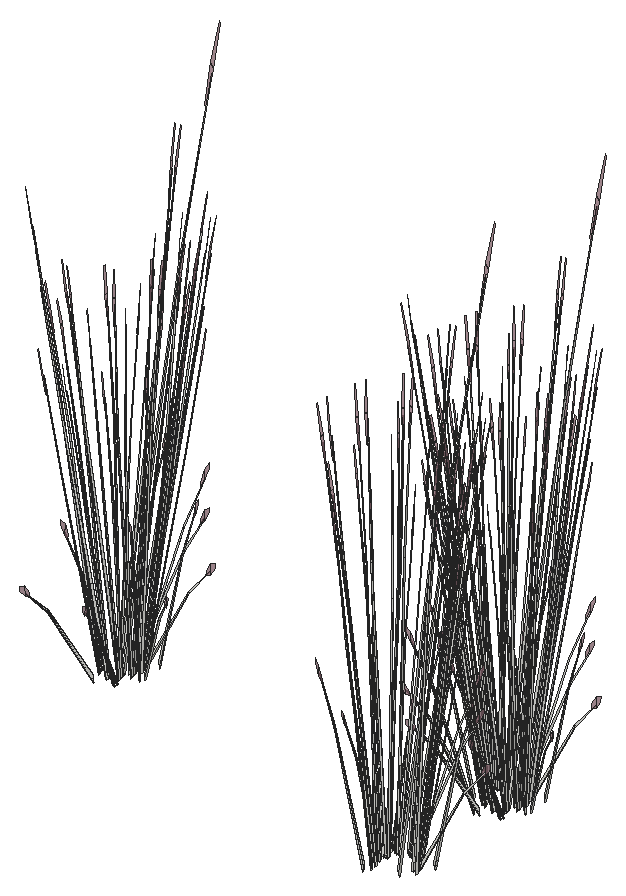
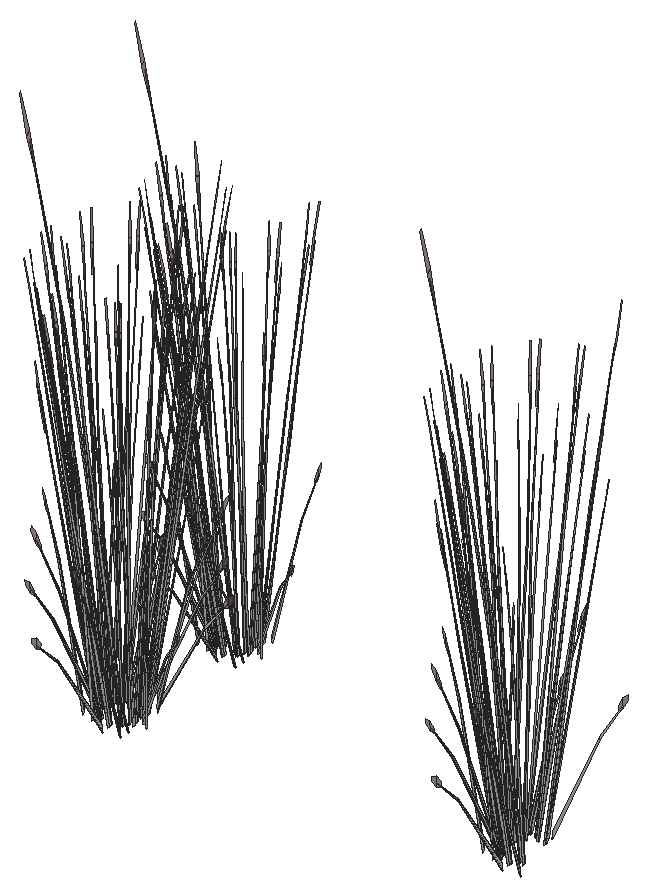
# SketchUp Ruby script. Lengths in inches.
U = 1.inch
M = Sketchup.active_model
def pt(a) = Geom::Point3d.new(a.map { |v| v * U })
def face(e, loops, mat)
  f = e.add_face(loops[0].map { |a| pt(a) })
  loops[1..].each { |l| e.add_face(l.map { |a| pt(a) }).erase! }
  f.material = f.back_material = mat if mat
  f
end
# faces: each face lists its corners as indices into pts; further lists are holes
def faces(e, pts, list, mat = nil) = list.each { |f| face(e, (f[0].is_a?(Array) ? f : [f]).map { |l| l.map { |i| pts[i] } }, mat) }
# xy, xz, yz: faces in a plane at the given z, y or x. An outline is a flat list of corners, or four numbers for a rectangle; further outlines are holes
def ring(l) = l.size == 4 ? [[l[0], l[1]], [l[2], l[1]], [l[2], l[3]], [l[0], l[3]]] : l.each_slice(2).to_a
def flat(e, list, mat, &to3) = list.each { |f| face(e, (f[0].is_a?(Array) ? f : [f]).map { |l| ring(l).map { |u, v| to3.(u, v) } }, mat) }
def xy(e, z, list, mat = nil) = flat(e, list, mat) { |x, y| [x, y, z] }
def xz(e, y, list, mat = nil) = flat(e, list, mat) { |x, z| [x, y, z] }
def yz(e, x, list, mat = nil) = flat(e, list, mat) { |y, z| [x, y, z] }
def lines(e, pts, list) = list.each { |a, b| e.add_line(pt(pts[a]), pt(pts[b])) }
# prism: a flat outline (further loops are holes) pulled along v
def prism(e, loops, v, mat = nil)
  f = face(e, loops, mat); d = Geom::Vector3d.new(v.map { |x| x * U })
  f.pushpull(f.normal.samedirection?(d) ? d.length : -d.length)
end
def box(e, o, s, mat = nil) = prism(e, [[o, [o[0] + s[0], o[1], o[2]], [o[0] + s[0], o[1] + s[1], o[2]], [o[0], o[1] + s[1], o[2]]]], [0, 0, s[2]], mat)
def at(x, y, z, deg = 0) = Geom::Transformation.translation(pt([x, y, z])) * Geom::Transformation.rotation(ORIGIN, Z_AXIS, deg.degrees)
def axes(o, x, y, z) = Geom::Transformation.new([*x, 0, *y, 0, *z, 0, *pt(o).to_a, 1])
def part(name) = M.definitions.add(name)
# library, detail: a bought-in or finely detailed component or shape, given as its bounding box
def library(name, o, s) = part(name).tap { |d| box(d.entities, o, s) }
def detail(e, o, s) = box(e.add_group.entities, o, s)
def put(e, d, t, mat = nil) = e.add_instance(d, t).tap { |i| i.material = mat if mat }
def group(e, t, mat = nil) = e.add_group.tap { |g| g.transformation = t; g.material = mat if mat }.entities
root = M.entities
M.materials.add("LightPink_Translucent").color = [144, 107, 117]
M.materials["LightPink_Translucent"].alpha = 0.75
c1 = part("blade")
p = [[2.15,0.21,22],[0,0.17,0],[0.09,0.45,0],[2.18,0.31,22],[2.29,0.31,22],[0.38,0.45,0],
  [2.48,0.24,33],[2.49,0.24,33],[2.48,0.22,33]]
faces(c1.entities,p,[[0,1,2,3],[4,5,2,3],[6,3,4,7],[8,0,3,6]])
c2 = part("seeds")
p = [[0.3,-0.1,1.38],[-0.01,-0.03,1.59],[-0.01,-0.03,0.03],[0.14,-0.07,-0.07],[0.29,-0.03,3],[0.15,0.01,3.11]]
faces(c2.entities,p,[[0,1,2,3],[1,0,4,5]],"LightPink_Translucent")
c3 = part("blade with seeds")
put(c3.entities,c1,at(0,0,0))
put(c3.entities,c2,axes([2.4,0.25,30.99],[1.5799,-0.05474,1.17369],[-0.12525,1.92788,0.29478],[-0.07173,-0.02425,1.56792]))
put(root,c3,axes([366.93,790.19,4.73],[-0.29004,-0.02173,0.0643],[0.00795,-0.32812,0.50621],[-0.03035,0.12569,0.77189]))
put(root,c3,axes([367.63,786.97,5.05],[0.05451,0.37564,0.35414],[-0.31161,0.09919,-0.4572],[-0.0837,-0.10765,0.87481]))
put(root,c3,axes([366.17,791.1875,4.71],[0.04004,-0.02816,1.77383],[0.33095,0.18728,-0.16761],[-0.00778,0.15594,0.31391]))
put(root,c3,axes([367.49,786.53,5.09],[0.39316,-0.11987,0.53763],[0.06823,0.47021,0.4433],[-0.09247,-0.13858,1.11249]))
put(root,c3,axes([367.58,786.63,4.73],[0.16041,-0.29625,0.0643],[0.22843,0.17248,0.50621],[-0.07385,-0.09498,0.77189]))
put(root,c3,axes([367.94,785.75,4.72],[-0.05398,-0.06539,1.74944],[-0.36026,0.04145,-0.27667],[-0.0575,-0.15639,0.14031]))
put(root,c3,axes([367.15,789.97,5.05],[0.23881,-0.24554,0.35414],[0.22606,0.28036,-0.4572],[-0.0344,0.14245,0.87481]))
put(root,c3,axes([366.99,790.03,5.4],[0.3879,0.02311,-0.13498],[-0.0106,0.43749,-0.74919],[-0.02694,0.1685,1.13838]))
put(root,c3,axes([368.48,786.76,5.03],[-0.34538,0.21713,-0.1216],[-0.16972,-0.38536,-0.67495],[-0.04557,-0.16239,1.02557]))
put(root,c3,axes([368.38,786.91,5.05],[-0.1064,0.35863,0.35414],[-0.31043,-0.1046,-0.4572],[-0.02846,-0.14439,0.87481]))
put(root,c3,axes([367.8125,790.67,5.0625],[-0.34777,-0.12192,0.53283],[0.11892,-0.40083,0.43934],[0.0209,0.15763,1.10256]))
put(root,c3,axes([367.72,790.7,4.73],[-0.26007,0.1585,0.0643],[-0.12729,-0.28902,0.50621],[0.02512,0.1274,0.77189]))
put(root,c3,axes([368.48,786.59,4.73],[0.26007,-0.1585,0.0643],[0.12729,0.28902,0.50621],[-0.02512,-0.1274,0.77189]))
put(root,c3,axes([367.63,791.38,4.72],[0.04474,0.0751,1.74944],[0.36104,0.0295,-0.27667],[0.03631,0.16562,0.14031]))
put(root,c3,axes([368.38,786.62,4.73],[0.34777,0.12192,0.48003],[-0.11892,0.40083,0.3958],[-0.0209,-0.15763,0.9933]))
put(root,c3,axes([367.82,790.37,5.05],[0.1064,-0.35863,0.35414],[0.31043,0.1046,-0.4572],[0.02846,0.14439,0.87481]))
put(root,c3,axes([368.23,791.65,5.65],[0.2439,-0.26754,-0.06488],[0.22348,0.29302,-0.29416],[0.01573,0.08303,0.97024]))
put(root,c3,axes([367.71,790.52,5.03],[0.34538,-0.21713,-0.1216],[0.16972,0.38536,-0.67495],[0.04557,0.16239,1.02557]))
put(root,c3,axes([369.48,786.22,4.71],[-0.03584,0.03562,1.77383],[-0.35118,-0.12018,-0.16761],[-0.01271,-0.15545,0.31391]))
put(root,c3,axes([369.2,787.25,5.03],[-0.3879,-0.02311,-0.1216],[0.0106,-0.43749,-0.67495],[0.02694,-0.1685,1.02557]))
put(root,c3,axes([369.05,787.32,5.05],[-0.23881,0.24554,0.35414],[-0.22606,-0.28036,-0.4572],[0.0344,-0.14245,0.87481]))
put(root,c3,axes([368.68,790.57,4.73],[-0.35104,0.10702,0.48003],[-0.06092,-0.41983,0.3958],[0.08256,0.12373,0.9933]))
put(root,c3,axes([368.61,790.65,4.73],[-0.16041,0.29625,0.0643],[-0.22843,-0.17248,0.50621],[0.07385,0.09498,0.77189]))
put(root,c3,axes([368.5625,790.3125,5.05],[-0.05451,-0.37564,0.35414],[0.31161,-0.09919,-0.4572],[0.0837,0.10765,0.87481]))
put(root,c3,axes([368.77,788.15,4.47],[-0.30498,-0.24231,1.38283],[0.32203,-0.37727,0.59665],[0.0984,0.22736,1.33663]))
put(root,c3,axes([368.26,790.84,4.71],[0.00104,-0.05646,1.77383],[0.30246,-0.2491,-0.16761],[0.10506,0.08891,0.31391]))
put(root,c3,axes([369.27,787.09,4.73],[0.29004,0.02173,0.0643],[-0.00795,0.32812,0.50621],[0.03035,-0.12569,0.77189]))
put(root,c3,axes([369.55,786.55,4.72],[-0.00341,-0.09282,1.74944],[-0.28775,-0.26825,-0.27667],[0.04449,-0.16261,0.14031]))
put(root,c3,axes([369.17,787.0625,4.73],[0.25132,0.3182,0.48003],[-0.2669,0.27442,0.3958],[0.04636,-0.14929,0.9933]))
put(root,c3,axes([369.46,788.07,5.05],[-0.30722,0.06665,0.35414],[-0.08112,-0.381,-0.4572],[0.08804,-0.10234,0.87481]))
put(root,c3,axes([368.53,790.51,5.03],[0.21031,-0.39918,-0.1216],[0.30457,0.22997,-0.67495],[0.10587,0.11278,1.02557]))
put(root,c3,axes([369.62,788.11,5.03],[-0.32648,-0.25715,-0.1216],[0.18809,-0.3724,-0.67495],[0.09224,-0.12945,1.02557]))
put(root,c3,axes([369.18,789.8,5.05],[-0.20082,-0.29199,0.35414],[0.2293,-0.2764,-0.4572],[0.1165,0.04206,0.87481]))
put(root,c3,axes([369.36,790.07,4.73],[-0.01777,0.35463,0.0643],[-0.26836,-0.00972,0.50621],[0.1028,0.03711,0.77189]))
put(root,c3,axes([369.39,789.96,4.73],[-0.26024,0.30729,0.48003],[-0.22444,-0.32634,0.3958],[0.1221,0.05668,0.9933]))
put(root,c3,axes([369.51,788.99,5.05],[-0.29332,-0.1301,0.35414],[0.08555,-0.37955,-0.4572],[0.11809,-0.0348,0.87481]))
put(root,c3,axes([369.74,788.01,4.73],[0.2423,0.19613,0.0643],[-0.14107,0.2793,0.50621],[0.07768,-0.0903,0.77189]))
put(root,c3,axes([369.67,787.93,4.73],[0.08753,0.42921,0.48003],[-0.34336,0.07449,0.3958],[0.1012,-0.10094,0.9933]))
put(root,c3,axes([370.43,788,4.71],[-0.0461,-0.00354,1.77383],[-0.19143,-0.37951,-0.16761],[0.07688,-0.12478,0.31391]))
put(root,c3,axes([369.78,789.1,4.73],[0.12963,0.31798,0.0643],[-0.23638,0.15564,0.50621],[0.1042,-0.03071,0.77189]))
put(root,c3,axes([369.24,789.99,5.03],[0.0189,-0.47427,-0.1216],[0.35781,0.01296,-0.67495],[0.13781,0.03295,1.02557]))
put(root,c3,axes([369.64,789.11,5.03],[-0.17758,-0.42229,-0.1216],[0.31518,-0.20752,-0.67495],[0.13282,-0.05572,1.02557]))
put(root,c3,axes([369.75,788.99,4.73],[-0.09971,0.42522,0.48003],[-0.32782,-0.1454,0.3958],[0.12892,-0.02555,0.9933]))
put(root,c3,axes([369.55,789.71,4.72],[0.07571,-0.00789,1.74944],[0.20767,-0.36231,-0.27667],[0.13467,0.04783,0.14031]))
put(root,c3,axes([370.34,790.37,4.71],[-0.03191,-0.04083,1.77383],[0.06981,-0.43764,-0.16761],[0.12571,-0.02796,0.31391]))
put(root,c3,axes([370.6,788.45,4.72],[0.04898,-0.07104,1.74944],[-0.06269,-0.43574,-0.27667],[0.12289,-0.08262,0.14031]))
put(root,c3,axes([400.14,777.88,4.72],[-0.05763,0.06055,1.74944],[0.0049,0.44239,-0.27667],[-0.13211,0.05753,0.14031]))
put(root,c3,axes([400.14,790.65,4.72],[-0.05763,0.06055,1.74944],[0.0049,0.44239,-0.27667],[-0.13211,0.05753,0.14031]))
put(root,c3,axes([399.5,778.33,4.71],[0.04504,0.01251,1.77383],[0.13934,0.41205,-0.16761],[-0.0922,0.10815,0.31391]))
put(root,c3,axes([399.5,791.1,4.71],[0.04504,0.01251,1.77383],[0.13934,0.41205,-0.16761],[-0.0922,0.10815,0.31391]))
put(root,c3,axes([400.42,776.04,4.71],[0.02617,0.04654,1.77383],[-0.12614,0.41836,-0.16761],[-0.12775,0.00303,0.31391]))
put(root,c3,axes([400.42,788.81,4.71],[0.02617,0.04654,1.77383],[-0.12614,0.41836,-0.16761],[-0.12775,0.00303,0.31391]))
put(root,c3,axes([400.71,788.53,4.72],[-0.07594,-0.00329,1.74944],[-0.24177,0.32918,-0.27667],[-0.129,-0.06726,0.14031]))
put(root,c3,axes([400.4,777.58,4.73],[0.09971,-0.42522,0.48003],[0.32782,0.1454,0.3958],[-0.12892,0.02555,0.9933]))
put(root,c3,axes([400.4,790.35,4.73],[0.09971,-0.42522,0.48003],[0.32782,0.1454,0.3958],[-0.12892,0.02555,0.9933]))
put(root,c3,axes([400.51,777.46,5.03],[0.17758,0.42229,-0.1216],[-0.31518,0.20752,-0.67495],[-0.13282,0.05572,1.02557]))
put(root,c3,axes([400.51,790.23,5.03],[0.17758,0.42229,-0.1216],[-0.31518,0.20752,-0.67495],[-0.13282,0.05572,1.02557]))
put(root,c3,axes([400.91,776.58,5.03],[-0.0189,0.47427,-0.1216],[-0.35781,-0.01296,-0.67495],[-0.13781,-0.03295,1.02557]))
put(root,c3,axes([400.91,789.35,5.03],[-0.0189,0.47427,-0.1216],[-0.35781,-0.01296,-0.67495],[-0.13781,-0.03295,1.02557]))
put(root,c3,axes([400.37,777.47,4.73],[-0.12963,-0.31798,0.0643],[0.23638,-0.15564,0.50621],[-0.1042,0.03071,0.77189]))
put(root,c3,axes([400.37,790.24,4.73],[-0.12963,-0.31798,0.0643],[0.23638,-0.15564,0.50621],[-0.1042,0.03071,0.77189]))
put(root,c3,axes([400.47,778.64,4.73],[-0.08753,-0.42921,0.48003],[0.34336,-0.07449,0.3958],[-0.1012,0.10094,0.9933]))
put(root,c3,axes([400.47,791.41,4.73],[-0.08753,-0.42921,0.48003],[0.34336,-0.07449,0.3958],[-0.1012,0.10094,0.9933]))
put(root,c3,axes([400.65,789.27,5.09],[0.29147,-0.34417,0.53763],[0.25138,0.3655,0.4433],[-0.13675,-0.06349,1.11249]))
put(root,c3,axes([400.41,778.56,4.73],[-0.2423,-0.19613,0.0643],[0.14107,-0.2793,0.50621],[-0.07768,0.0903,0.77189]))
put(root,c3,axes([400.41,791.33,4.73],[-0.2423,-0.19613,0.0643],[0.14107,-0.2793,0.50621],[-0.07768,0.0903,0.77189]))
put(root,c3,axes([400.64,777.59,5.05],[0.29332,0.1301,0.35414],[-0.08555,0.37955,-0.4572],[-0.11809,0.0348,0.87481]))
put(root,c3,axes([400.64,790.35,5.05],[0.29332,0.1301,0.35414],[-0.08555,0.37955,-0.4572],[-0.11809,0.0348,0.87481]))
put(root,c3,axes([400.78,789.27,4.73],[0.01777,-0.35463,0.0643],[0.26836,0.00972,0.50621],[-0.1028,-0.03711,0.77189]))
put(root,c3,axes([400.15,779.53,4.72],[-0.00877,0.09229,1.74944],[0.24897,0.32105,-0.27667],[-0.06518,0.15182,0.14031]))
put(root,c3,axes([400.15,792.3,4.72],[-0.00877,0.09229,1.74944],[0.24897,0.32105,-0.27667],[-0.06518,0.15182,0.14031]))
put(root,c3,axes([401.61,788.66,5.43],[-0.23555,0.44708,-0.13619],[-0.34112,-0.25757,-0.75594],[-0.11858,-0.12631,1.14864]))
put(root,c3,axes([400.97,776.77,5.05],[0.20082,0.29199,0.35414],[-0.2293,0.2764,-0.4572],[-0.1165,-0.04206,0.87481]))
put(root,c3,axes([400.97,789.54,5.05],[0.20082,0.29199,0.35414],[-0.2293,0.2764,-0.4572],[-0.1165,-0.04206,0.87481]))
put(root,c3,axes([400.53,778.46,5.03],[0.32648,0.25715,-0.1216],[-0.18809,0.3724,-0.67495],[-0.09224,0.12945,1.02557]))
put(root,c3,axes([400.53,791.23,5.03],[0.32648,0.25715,-0.1216],[-0.18809,0.3724,-0.67495],[-0.09224,0.12945,1.02557]))
put(root,c3,axes([399.99,779.58,5.65],[0.31145,0.12449,-0.06488],[-0.0958,0.38314,-0.29416],[-0.05094,0.05817,0.97024]))
put(root,c3,axes([399.99,792.35,5.65],[0.31145,0.12449,-0.06488],[-0.0958,0.38314,-0.29416],[-0.05094,0.05817,0.97024]))
put(root,c3,axes([400.6875,778.5,5.05],[0.30722,-0.06665,0.35414],[0.08112,0.381,-0.4572],[-0.08804,0.10234,0.87481]))
put(root,c3,axes([400.6875,791.27,5.05],[0.30722,-0.06665,0.35414],[0.08112,0.381,-0.4572],[-0.08804,0.10234,0.87481]))
put(root,c3,axes([401.52,787.59,4.71],[-0.00658,0.0559,1.77383],[-0.32474,0.20287,-0.16761],[-0.09556,-0.1037,0.31391]))
put(root,c3,axes([400.98,779.51,4.73],[-0.25132,-0.3182,0.48003],[0.2669,-0.27442,0.3958],[-0.04636,0.14929,0.9933]))
put(root,c3,axes([400.98,792.28,4.73],[-0.25132,-0.3182,0.48003],[0.2669,-0.27442,0.3958],[-0.04636,0.14929,0.9933]))
put(root,c3,axes([400.88,779.48,4.73],[-0.29004,-0.02173,0.0643],[0.00795,-0.32812,0.50621],[-0.03035,0.12569,0.77189]))
put(root,c3,axes([400.88,792.25,4.73],[-0.29004,-0.02173,0.0643],[0.00795,-0.32812,0.50621],[-0.03035,0.12569,0.77189]))
put(root,c3,axes([401.59,789.03,5.05],[0.05451,0.37564,0.35414],[-0.31161,0.09919,-0.4572],[-0.0837,-0.10765,0.87481]))
put(root,c3,axes([400.125,780.48,4.71],[0.04004,-0.02816,1.77383],[0.33095,0.18728,-0.16761],[-0.00778,0.15594,0.31391]))
put(root,c3,axes([400.125,793.25,4.71],[0.04004,-0.02816,1.77383],[0.33095,0.18728,-0.16761],[-0.00778,0.15594,0.31391]))
put(root,c3,axes([401.45,788.59,5.09],[0.39316,-0.11987,0.53763],[0.06823,0.47021,0.4433],[-0.09247,-0.13858,1.11249]))
put(root,c3,axes([401.54,788.6875,4.73],[0.16041,-0.29625,0.0643],[0.22843,0.17248,0.50621],[-0.07385,-0.09498,0.77189]))
put(root,c3,axes([401.89,787.81,4.72],[-0.05398,-0.06539,1.74944],[-0.36026,0.04145,-0.27667],[-0.0575,-0.15639,0.14031]))
put(root,c3,axes([401.1,779.26,5.05],[0.23881,-0.24554,0.35414],[0.22606,0.28036,-0.4572],[-0.0344,0.14245,0.87481]))
put(root,c3,axes([401.1,792.02,5.05],[0.23881,-0.24554,0.35414],[0.22606,0.28036,-0.4572],[-0.0344,0.14245,0.87481]))
put(root,c3,axes([400.95,779.32,5.4],[0.3879,0.02311,-0.13498],[-0.0106,0.43749,-0.74919],[-0.02694,0.1685,1.13838]))
put(root,c3,axes([400.95,792.09,5.4],[0.3879,0.02311,-0.13498],[-0.0106,0.43749,-0.74919],[-0.02694,0.1685,1.13838]))
put(root,c3,axes([402.4375,788.82,5.03],[-0.34538,0.21713,-0.1216],[-0.16972,-0.38536,-0.67495],[-0.04557,-0.16239,1.02557]))
put(root,c3,axes([402.33,788.97,5.05],[-0.1064,0.35863,0.35414],[-0.31043,-0.1046,-0.4572],[-0.02846,-0.14439,0.87481]))
put(root,c3,axes([401.77,779.95,5.0625],[-0.34777,-0.12192,0.53283],[0.11892,-0.40083,0.43934],[0.0209,0.15763,1.10256]))
put(root,c3,axes([401.77,792.72,5.0625],[-0.34777,-0.12192,0.53283],[0.11892,-0.40083,0.43934],[0.0209,0.15763,1.10256]))
put(root,c3,axes([401.67,779.98,4.73],[-0.26007,0.1585,0.0643],[-0.12729,-0.28902,0.50621],[0.02512,0.1274,0.77189]))
put(root,c3,axes([401.67,792.75,4.73],[-0.26007,0.1585,0.0643],[-0.12729,-0.28902,0.50621],[0.02512,0.1274,0.77189]))
put(root,c3,axes([402.43,788.64,4.73],[0.26007,-0.1585,0.0643],[0.12729,0.28902,0.50621],[-0.02512,-0.1274,0.77189]))
put(root,c3,axes([401.58,780.67,4.72],[0.04474,0.0751,1.74944],[0.36104,0.0295,-0.27667],[0.03631,0.16562,0.14031]))
put(root,c3,axes([401.58,793.44,4.72],[0.04474,0.0751,1.74944],[0.36104,0.0295,-0.27667],[0.03631,0.16562,0.14031]))
put(root,c3,axes([402.34,788.67,4.73],[0.34777,0.12192,0.48003],[-0.11892,0.40083,0.3958],[-0.0209,-0.15763,0.9933]))
put(root,c3,axes([401.77,779.66,5.05],[0.1064,-0.35863,0.35414],[0.31043,0.1046,-0.4572],[0.02846,0.14439,0.87481]))
put(root,c3,axes([401.77,792.43,5.05],[0.1064,-0.35863,0.35414],[0.31043,0.1046,-0.4572],[0.02846,0.14439,0.87481]))
put(root,c3,axes([402.1875,780.9375,5.65],[0.2439,-0.26754,-0.06488],[0.22348,0.29302,-0.29416],[0.01573,0.08303,0.97024]))
put(root,c3,axes([402.1875,793.71,5.65],[0.2439,-0.26754,-0.06488],[0.22348,0.29302,-0.29416],[0.01573,0.08303,0.97024]))
put(root,c3,axes([401.67,779.81,5.03],[0.34538,-0.21713,-0.1216],[0.16972,0.38536,-0.67495],[0.04557,0.16239,1.02557]))
put(root,c3,axes([401.67,792.58,5.03],[0.34538,-0.21713,-0.1216],[0.16972,0.38536,-0.67495],[0.04557,0.16239,1.02557]))
put(root,c3,axes([403.43,788.28,4.71],[-0.03584,0.03562,1.77383],[-0.35118,-0.12018,-0.16761],[-0.01271,-0.15545,0.31391]))
put(root,c3,axes([403.15,789.31,5.03],[-0.3879,-0.02311,-0.1216],[0.0106,-0.43749,-0.67495],[0.02694,-0.1685,1.02557]))
put(root,c3,axes([403,789.37,5.05],[-0.23881,0.24554,0.35414],[-0.22606,-0.28036,-0.4572],[0.0344,-0.14245,0.87481]))
put(root,c3,axes([402.63,779.86,4.73],[-0.35104,0.10702,0.48003],[-0.06092,-0.41983,0.3958],[0.08256,0.12373,0.9933]))
put(root,c3,axes([402.63,792.625,4.73],[-0.35104,0.10702,0.48003],[-0.06092,-0.41983,0.3958],[0.08256,0.12373,0.9933]))
put(root,c3,axes([402.56,779.94,4.73],[-0.16041,0.29625,0.0643],[-0.22843,-0.17248,0.50621],[0.07385,0.09498,0.77189]))
put(root,c3,axes([402.56,792.71,4.73],[-0.16041,0.29625,0.0643],[-0.22843,-0.17248,0.50621],[0.07385,0.09498,0.77189]))
put(root,c3,axes([402.52,779.6,5.05],[-0.05451,-0.37564,0.35414],[0.31161,-0.09919,-0.4572],[0.0837,0.10765,0.87481]))
put(root,c3,axes([402.52,792.37,5.05],[-0.05451,-0.37564,0.35414],[0.31161,-0.09919,-0.4572],[0.0837,0.10765,0.87481]))
put(root,c3,axes([402.72,777.4375,4.47],[-0.30498,-0.24231,1.38283],[0.32203,-0.37727,0.59665],[0.0984,0.22736,1.33663]))
put(root,c3,axes([402.72,790.21,4.47],[-0.30498,-0.24231,1.38283],[0.32203,-0.37727,0.59665],[0.0984,0.22736,1.33663]))
put(root,c3,axes([402.21,780.125,4.71],[0.00104,-0.05646,1.77383],[0.30246,-0.2491,-0.16761],[0.10506,0.08891,0.31391]))
put(root,c3,axes([402.21,792.89,4.71],[0.00104,-0.05646,1.77383],[0.30246,-0.2491,-0.16761],[0.10506,0.08891,0.31391]))
put(root,c3,axes([403.22,789.15,4.73],[0.29004,0.02173,0.0643],[-0.00795,0.32812,0.50621],[0.03035,-0.12569,0.77189]))
put(root,c3,axes([403.51,788.61,4.72],[-0.00341,-0.09282,1.74944],[-0.28775,-0.26825,-0.27667],[0.04449,-0.16261,0.14031]))
put(root,c3,axes([403.125,789.12,4.73],[0.25132,0.3182,0.48003],[-0.2669,0.27442,0.3958],[0.04636,-0.14929,0.9933]))
put(root,c3,axes([403.42,790.13,5.05],[-0.30722,0.06665,0.35414],[-0.08112,-0.381,-0.4572],[0.08804,-0.10234,0.87481]))
put(root,c3,axes([402.49,779.79,5.03],[0.21031,-0.39918,-0.1216],[0.30457,0.22997,-0.67495],[0.10587,0.11278,1.02557]))
put(root,c3,axes([402.49,792.5625,5.03],[0.21031,-0.39918,-0.1216],[0.30457,0.22997,-0.67495],[0.10587,0.11278,1.02557]))
put(root,c3,axes([403.58,790.17,5.03],[-0.32648,-0.25715,-0.1216],[0.18809,-0.3724,-0.67495],[0.09224,-0.12945,1.02557]))
put(root,c3,axes([403.14,779.09,5.05],[-0.20082,-0.29199,0.35414],[0.2293,-0.2764,-0.4572],[0.1165,0.04206,0.87481]))
put(root,c3,axes([403.14,791.86,5.05],[-0.20082,-0.29199,0.35414],[0.2293,-0.2764,-0.4572],[0.1165,0.04206,0.87481]))
put(root,c3,axes([403.32,779.36,4.73],[-0.01777,0.35463,0.0643],[-0.26836,-0.00972,0.50621],[0.1028,0.03711,0.77189]))
put(root,c3,axes([403.32,792.125,4.73],[-0.01777,0.35463,0.0643],[-0.26836,-0.00972,0.50621],[0.1028,0.03711,0.77189]))
put(root,c3,axes([403.34,779.24,4.73],[-0.26024,0.30729,0.48003],[-0.22444,-0.32634,0.3958],[0.1221,0.05668,0.9933]))
put(root,c3,axes([403.34,792.01,4.73],[-0.26024,0.30729,0.48003],[-0.22444,-0.32634,0.3958],[0.1221,0.05668,0.9933]))
put(root,c3,axes([403.47,778.27,5.05],[-0.29332,-0.1301,0.35414],[0.08555,-0.37955,-0.4572],[0.11809,-0.0348,0.87481]))
put(root,c3,axes([403.47,791.04,5.05],[-0.29332,-0.1301,0.35414],[0.08555,-0.37955,-0.4572],[0.11809,-0.0348,0.87481]))
put(root,c3,axes([403.7,790.07,4.73],[0.2423,0.19613,0.0643],[-0.14107,0.2793,0.50621],[0.07768,-0.0903,0.77189]))
put(root,c3,axes([403.63,789.99,4.73],[0.08753,0.42921,0.48003],[-0.34336,0.07449,0.3958],[0.1012,-0.10094,0.9933]))
put(root,c3,axes([404.38,790.05,4.71],[-0.0461,-0.00354,1.77383],[-0.19143,-0.37951,-0.16761],[0.07688,-0.12478,0.31391]))
put(root,c3,axes([403.73,778.39,4.73],[0.12963,0.31798,0.0643],[-0.23638,0.15564,0.50621],[0.1042,-0.03071,0.77189]))
put(root,c3,axes([403.73,791.16,4.73],[0.12963,0.31798,0.0643],[-0.23638,0.15564,0.50621],[0.1042,-0.03071,0.77189]))
put(root,c3,axes([403.19,779.28,5.03],[0.0189,-0.47427,-0.1216],[0.35781,0.01296,-0.67495],[0.13781,0.03295,1.02557]))
put(root,c3,axes([403.19,792.05,5.03],[0.0189,-0.47427,-0.1216],[0.35781,0.01296,-0.67495],[0.13781,0.03295,1.02557]))
put(root,c3,axes([403.59,778.4,5.03],[-0.17758,-0.42229,-0.1216],[0.31518,-0.20752,-0.67495],[0.13282,-0.05572,1.02557]))
put(root,c3,axes([403.59,791.17,5.03],[-0.17758,-0.42229,-0.1216],[0.31518,-0.20752,-0.67495],[0.13282,-0.05572,1.02557]))
put(root,c3,axes([403.71,778.28,4.73],[-0.09971,0.42522,0.48003],[-0.32782,-0.1454,0.3958],[0.12892,-0.02555,0.9933]))
put(root,c3,axes([403.71,791.05,4.73],[-0.09971,0.42522,0.48003],[-0.32782,-0.1454,0.3958],[0.12892,-0.02555,0.9933]))
put(root,c3,axes([403.5,778.99,4.72],[0.07571,-0.00789,1.74944],[0.20767,-0.36231,-0.27667],[0.13467,0.04783,0.14031]))
put(root,c3,axes([403.5,791.76,4.72],[0.07571,-0.00789,1.74944],[0.20767,-0.36231,-0.27667],[0.13467,0.04783,0.14031]))
put(root,c3,axes([404.3,779.66,4.71],[-0.03191,-0.04083,1.77383],[0.06981,-0.43764,-0.16761],[0.12571,-0.02796,0.31391]))
put(root,c3,axes([404.3,792.42,4.71],[-0.03191,-0.04083,1.77383],[0.06981,-0.43764,-0.16761],[0.12571,-0.02796,0.31391]))
put(root,c3,axes([404.55,790.51,4.72],[0.04898,-0.07104,1.74944],[-0.06269,-0.43574,-0.27667],[0.12289,-0.08262,0.14031]))
